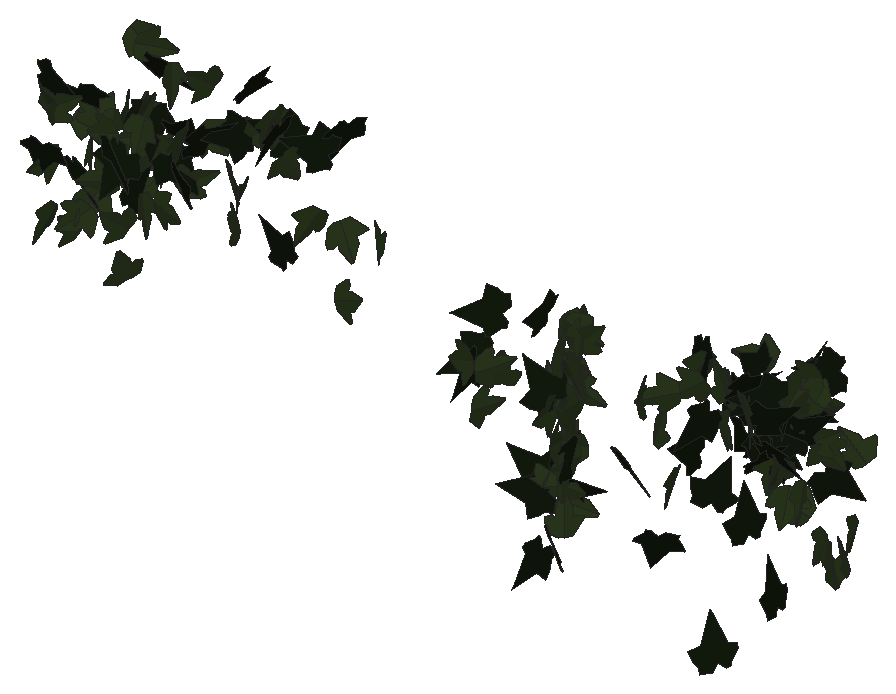
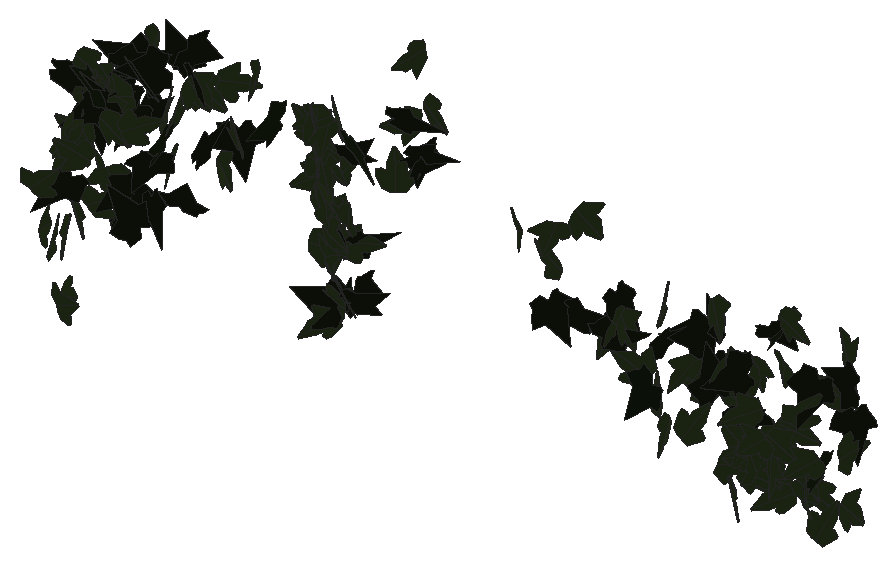
# SketchUp Ruby script. Lengths in inches.
U = 1.inch
M = Sketchup.active_model
def pt(a) = Geom::Point3d.new(a.map { |v| v * U })
def face(e, loops, mat)
  f = e.add_face(loops[0].map { |a| pt(a) })
  loops[1..].each { |l| e.add_face(l.map { |a| pt(a) }).erase! }
  f.material = f.back_material = mat if mat
  f
end
# faces: each face lists its corners as indices into pts; further lists are holes
def faces(e, pts, list, mat = nil) = list.each { |f| face(e, (f[0].is_a?(Array) ? f : [f]).map { |l| l.map { |i| pts[i] } }, mat) }
# xy, xz, yz: faces in a plane at the given z, y or x. An outline is a flat list of corners, or four numbers for a rectangle; further outlines are holes
def ring(l) = l.size == 4 ? [[l[0], l[1]], [l[2], l[1]], [l[2], l[3]], [l[0], l[3]]] : l.each_slice(2).to_a
def flat(e, list, mat, &to3) = list.each { |f| face(e, (f[0].is_a?(Array) ? f : [f]).map { |l| ring(l).map { |u, v| to3.(u, v) } }, mat) }
def xy(e, z, list, mat = nil) = flat(e, list, mat) { |x, y| [x, y, z] }
def xz(e, y, list, mat = nil) = flat(e, list, mat) { |x, z| [x, y, z] }
def yz(e, x, list, mat = nil) = flat(e, list, mat) { |y, z| [x, y, z] }
def lines(e, pts, list) = list.each { |a, b| e.add_line(pt(pts[a]), pt(pts[b])) }
# prism: a flat outline (further loops are holes) pulled along v
def prism(e, loops, v, mat = nil)
  f = face(e, loops, mat); d = Geom::Vector3d.new(v.map { |x| x * U })
  f.pushpull(f.normal.samedirection?(d) ? d.length : -d.length)
end
def box(e, o, s, mat = nil) = prism(e, [[o, [o[0] + s[0], o[1], o[2]], [o[0] + s[0], o[1] + s[1], o[2]], [o[0], o[1] + s[1], o[2]]]], [0, 0, s[2]], mat)
def at(x, y, z, deg = 0) = Geom::Transformation.translation(pt([x, y, z])) * Geom::Transformation.rotation(ORIGIN, Z_AXIS, deg.degrees)
def axes(o, x, y, z) = Geom::Transformation.new([*x, 0, *y, 0, *z, 0, *pt(o).to_a, 1])
def part(name) = M.definitions.add(name)
# library, detail: a bought-in or finely detailed component or shape, given as its bounding box
def library(name, o, s) = part(name).tap { |d| box(d.entities, o, s) }
def detail(e, o, s) = box(e.add_group.entities, o, s)
def put(e, d, t, mat = nil) = e.add_instance(d, t).tap { |i| i.material = mat if mat }
def group(e, t, mat = nil) = e.add_group.tap { |g| g.transformation = t; g.material = mat if mat }.entities
root = M.entities
M.materials.add("efeu1").color = [18, 25, 13]
M.materials.add("efeu2").color = [43, 57, 29]
c1 = part("ivyleaf_10")
p = [[0,0.5,-0.03],[-0.0625,2.02,-0.43],[-0.19,2.01,-0.46],[-0.54,1.05,-0.29],[-0.52,0.625,-0.18],[-0.83,0.76,-0.28],
  [-1.16,0.64,-0.33],[-1.15,0.33,-0.24],[-0.77,-0.39,0.02],[-0.3,-0.51,0.16],[0.04,-0.48,0.23],[-0.02,2.01,-0.4375],
  [-0.06,2.01,-0.43],[0.04,-0.49,0.23],[0.67,-0.49,0.14],[1.38,0.36,-0.2],[1.375,0.51,-0.24],[0.81,0.65,-0.19],
  [0.62,0.59,-0.15],[0.6,1.09,-0.28],[0.5,1.23,-0.31]]
faces(c1.entities,p,[[0,1,2,3,4,5,6,7,8,9,10],[11,12,0,13,14,15,16,17,18,19,20]],"efeu2")
c2 = part("ivyleaf_9")
p = [[1.54,2.16,1.25],[1.36,2.04,1.19],[-0.21,0.99,0.68],[-0.71,1.11,0.82],[-0.85,0.86,0.67],[-0.8,0.17,0.21],
  [-0.9,-0.01,0.1],[-0.67,-0.16,-0.02],[-0.08,-0.08,-0.05],[-0.03,-0.6,-0.4],[0.65,-0.88,-0.66],[0.83,-0.6,-0.49],
  [1.29,-0.42,-0.43],[1.8125,-0.07,-0.26],[1.21,0.44,0.15]]
faces(c2.entities,p,[[0,1,2,3,4,5,6,7,8,9,10,11,12,13,14]],"efeu1")
put(root,c1,axes([26.62,223.76,193.08],[-0.0284,0.01779,-0.49888],[-0.14979,-0.47696,-0.00849],[-0.47619,0.14897,0.03242]))
put(root,c2,axes([26.15,223.96,195.55],[0.24856,-0.04735,-0.43125],[0.42245,0.13954,0.22817],[0.09874,-0.47779,0.10937]))
put(root,c1,axes([26.58,223.71,191.38],[0.07742,-0.36257,0.33548],[0.07667,-0.32664,-0.37071],[0.48798,0.10884,0.00502]))
put(root,c1,axes([26.34,225.81,192.59],[0.13191,-0.08299,0.47509],[0.38107,-0.28397,-0.15541],[0.29561,0.40308,-0.01167]))
put(root,c1,axes([26.45,225.41,193.65],[0.21774,0.18874,0.40861],[0.30341,0.27373,-0.28812],[-0.33246,0.37343,0.00467]))
put(root,c1,axes([26.47,227.7,195.32],[0.28749,0.11923,0.39132],[0.36164,0.1495,-0.31124],[-0.19122,0.46199,-0.00028]))
put(root,c2,axes([26.93,222.92,193.96],[0.29364,0.23583,-0.32887],[-0.27196,-0.1859,-0.37614],[-0.29968,0.39978,0.0191]))
put(root,c1,axes([27.04,224.35,190.71],[-0.1528,-0.2963,-0.37264],[-0.13276,-0.34932,0.33219],[-0.45719,0.20047,0.02808]))
put(root,c1,axes([26.73,223.62,194.81],[-0.25829,-0.13735,0.40549],[0.35117,0.20289,0.29242],[-0.24487,0.43585,-0.00834]))
put(root,c1,axes([27.13,226.38,193.78],[0.08231,-0.36855,-0.32771],[-0.08156,0.3175,-0.37755],[0.48639,0.11561,-0.00785]))
put(root,c2,axes([26.97,224.32,192.74],[0.34112,-0.36522,0.01576],[0.0134,-0.00904,-0.49974],[0.36532,0.34137,0.00362]))
put(root,c2,axes([27.3125,224.11,195.39],[0.39415,0.29152,-0.09829],[-0.07931,-0.05806,-0.49024],[-0.29725,0.40205,0.00047]))
put(root,c1,axes([27.53,224.75,194.38],[0.22778,0.33838,0.28916],[-0.15531,-0.24398,0.40786],[0.41713,-0.27562,-0.00604]))
put(root,c1,axes([27.64,223.89,191.63],[0.33009,0.08195,-0.36651],[-0.36287,-0.05617,-0.33937],[-0.0968,0.49003,0.02239]))
put(root,c1,axes([27.28,222.7,195.51],[-0.27672,0.06796,0.41086],[0.38661,-0.14143,0.28378],[0.15479,0.47474,0.02573]))
put(root,c1,axes([27.29,225.6,192.34],[0.09866,0.14487,0.46827],[0.27252,0.38083,-0.17523],[-0.40743,0.2898,-0.00381]))
put(root,c1,axes([27.41,226.92,195.62],[0.0891,0.08984,0.48372],[0.212,0.4366,-0.12014],[-0.44398,0.22651,0.03971]))
put(root,c1,axes([27.74,224.29,192.03],[0.28153,0.30283,-0.28112],[-0.20739,-0.19066,-0.41308],[-0.35739,0.3492,0.01825]))
put(root,c1,axes([28.02,226.3125,193.18],[0.15422,0.04089,-0.47386],[-0.47392,-0.02887,-0.15673],[-0.04018,0.49749,0.02985]))
put(root,c1,axes([27.72,226.32,193.34],[0.0667,0.42113,-0.26115],[0.04213,0.25773,0.42638],[0.49374,-0.07889,-0.0011]))
put(root,c1,axes([28.21,226.27,194.11],[-0.01737,0.40647,-0.29065],[0.00094,-0.2908,-0.40674],[-0.4997,-0.01468,0.00934]))
put(root,c1,axes([28.66,224.4,193.08],[-0.23568,-0.18544,0.40008],[-0.31994,-0.24028,-0.29984],[0.30347,-0.39734,-0.0054]))
put(root,c1,axes([28.73,223.69,193.18],[-0.10709,-0.05814,0.48492],[-0.41611,-0.24906,-0.12175],[0.2557,-0.42964,0.00496]))
put(root,c1,axes([28.64,226.32,192.53],[0.2734,-0.36018,-0.21337],[-0.12078,0.17613,-0.45209],[0.40083,0.29875,0.0093]))
put(root,c1,axes([28.62,225.48,193.18],[0.02432,0.08357,-0.49237],[0.19315,0.45301,0.08643],[0.46054,-0.19441,-0.01025]))
put(root,c1,axes([29,226.13,193.03],[0.11589,0.11121,-0.4735],[-0.33248,-0.33716,-0.16057],[-0.355,0.35207,-0.0042]))
put(root,c2,axes([28.74,225.58,194.55],[-0.2933,-0.32037,-0.24767],[0.17032,0.17985,-0.43433],[0.36738,-0.33915,0.00363]))
put(root,c2,axes([28.56,225.8125,195.9375],[0.45319,-0.05575,0.20375],[0.20116,-0.03326,-0.45654],[0.06446,0.49577,-0.00771]))
put(root,c1,axes([28.83,223.68,195.19],[0.42507,-0.15942,0.20952],[0.19549,-0.0754,-0.45398],[0.17634,0.46787,-0.00177]))
put(root,c1,axes([29.18,227.66,194.68],[-0.14249,-0.24996,-0.40892],[-0.20497,-0.35385,0.28771],[-0.43323,0.24962,-0.00163]))
put(root,c1,axes([29.2,224.58,194.89],[0.07486,-0.16035,0.46764],[-0.23222,0.40614,0.17644],[-0.43643,-0.2436,-0.01367]))
put(root,c1,axes([29.39,225.38,193.61],[0.29267,-0.08357,-0.39669],[-0.36996,0.145,-0.30349],[0.16577,0.47116,0.02304]))
put(root,c2,axes([29.13,224.09,192.4],[-0.19206,0.31082,0.34132],[0.1802,-0.28988,0.36537],[0.42502,0.26336,-0.00067]))
put(root,c1,axes([29.15,224.36,192.47],[0.36808,-0.0235,-0.33759],[0.33789,-0.00205,0.36855],[-0.01871,-0.49944,0.01437]))
put(root,c1,axes([29.4,225.67,196],[-0.03051,0.46685,-0.17641],[0.01122,-0.17605,-0.46785],[-0.49894,-0.0325,0.00027]))
put(root,c1,axes([29.85,222.3125,195.68],[0.18102,-0.08307,-0.45862],[-0.4215,0.1808,-0.19912],[0.19892,0.4587,-0.00457]))
put(root,c1,axes([29.7,223.14,192.25],[-0.17859,-0.24892,-0.39515],[-0.22572,-0.32435,0.30634],[-0.40885,0.2878,0.00348]))
put(root,c1,axes([29.66,223.97,195.13],[0.49312,-0.08109,-0.01608],[-0.01551,0.00484,-0.49974],[0.0812,0.49336,0.00226]))
put(root,c1,axes([29.8125,223.07,190.75],[-0.21269,-0.41069,-0.19],[-0.08712,-0.16885,0.46249],[-0.44404,0.22984,0.00027]))
put(root,c1,axes([30.21,223.38,193.08],[-0.11617,0.47045,-0.1232],[0.03003,-0.11949,-0.48458],[-0.48539,-0.11999,-0.00049]))
put(root,c2,axes([30.03,222.21,195.34],[0.23477,-0.43236,0.08915],[0.04009,-0.07968,-0.49198],[0.43963,0.23815,-0.00275]))
put(root,c2,axes([30.48,222.21,195.19],[-0.39779,-0.30206,-0.02288],[0.0212,0.00992,-0.49945],[0.30218,-0.39833,0.00491]))
put(root,c2,axes([30.1875,225.09,194.47],[0.49966,0.01557,-0.00997],[0.00951,0.01506,0.49968],[0.01586,-0.49953,0.01475]))
put(root,c2,axes([30.89,227.16,195.34],[0.12961,0.38678,0.28914],[0.09464,0.27322,-0.40791],[-0.47355,0.16046,-0.00238]))
put(root,c2,axes([30.94,223.71,194.66],[0.02144,-0.28482,-0.41039],[-0.03384,0.40899,-0.28562],[0.49839,0.04002,-0.00173]))
put(root,c1,axes([30.84,223.35,193.22],[-0.04714,0.02418,-0.49719],[0.42355,-0.26041,-0.05282],[-0.2615,-0.42615,0.00406]))
put(root,c1,axes([31.19,224.96,194.95],[0.0858,0.36591,0.32977],[0.08116,0.31966,-0.37581],[-0.48585,0.11802,-0.00454]))
put(root,c1,axes([31.34,225.88,193.34],[-0.36488,0.34077,0.02714],[-0.02135,0.0169,-0.49926],[-0.34118,-0.3655,0.00222]))
put(root,c1,axes([31.2,224.03,193.73],[-0.15654,-0.17991,0.43947],[0.2864,0.33333,0.23847],[-0.37878,0.32638,-0.00131]))
put(root,c1,axes([31.6875,223.25,195.86],[0.09218,-0.49118,-0.01556],[-0.00321,0.01523,-0.49976],[0.49142,0.09223,-0.00034]))
put(root,c2,axes([31.62,223.79,195.3],[0.03251,0.36527,-0.33989],[-0.02699,0.34139,0.36431],[0.49821,-0.00534,0.04191]))
put(root,c2,axes([32.27,225.23,195.25],[0.04968,-0.35318,-0.35043],[0.08062,-0.3418,0.35591],[-0.49095,-0.09186,0.02299]))
put(root,c2,axes([32.07,222.74,194.52],[-0.02639,-0.07411,0.49377],[0.2081,-0.4511,-0.05658],[0.45387,0.20252,0.05466]))
put(root,c1,axes([32.16,225.96,194.81],[-0.20519,-0.26163,0.37343],[0.23032,0.29394,0.33249],[-0.39351,0.30846,-0.00011]))
put(root,c1,axes([32.33,225.07,193.21],[0.11461,-0.35333,-0.33469],[0.09839,-0.31993,0.37144],[-0.47664,-0.151,-0.00381]))
put(root,c1,axes([33.08,225.57,195.9],[0.07329,-0.46972,0.15491],[0.04221,-0.15008,-0.47507],[0.49279,0.08272,0.01766]))
put(root,c2,axes([33.68,225.72,195.27],[-0.15169,0.03844,0.47488],[-0.47006,0.06916,-0.15574],[-0.07766,-0.4937,0.01515]))
put(root,c1,axes([33.3,225.78,195.91],[-0.00775,0.34917,-0.3578],[-0.00742,-0.35788,-0.34909],[-0.49988,-0.0001,0.01073]))
put(root,c2,axes([33.93,224.82,196.17],[-0.21053,0.35683,-0.2799],[0.12905,-0.2487,-0.41412],[-0.43477,-0.24662,0.01262]))
put(root,c1,axes([34.1,224.89,195.17],[-0.17733,-0.39408,-0.2515],[0.10974,0.22638,-0.4321],[0.45444,-0.20844,0.0062]))
put(root,c1,axes([34.39,222.3,194.17],[-0.25718,0.3059,0.30047],[0.19285,-0.23042,0.39964],[0.38297,0.32145,0.00053]))
put(root,c2,axes([35.04,225.56,195.4],[-0.22892,0.04265,0.44247],[-0.43705,0.06925,-0.23279],[-0.08114,-0.49334,0.00558]))
put(root,c2,axes([35.28,226.22,196.07],[-0.04527,0.36959,-0.33369],[0.05326,-0.32955,-0.37224],[-0.49509,-0.06925,-0.00953]))
put(root,c2,axes([35.59,223.03,193.35],[0.03167,-0.05461,0.496],[-0.34113,0.36035,0.06145],[-0.36418,-0.34229,-0.01444]))
put(root,c1,axes([37.73,221.71,196.01],[-0.12506,-0.37647,0.30435],[-0.05999,-0.29987,-0.39558],[0.48038,-0.13546,0.02983]))
put(root,c1,axes([38.35,222.16,195.6],[0.28487,0.38413,0.14592],[0.08768,0.11664,-0.47823],[-0.40145,0.29806,-0.00091]))
put(root,c1,axes([38.92,221.42,193.86],[0.15555,-0.10273,-0.46395],[0.40968,-0.21835,0.1857],[-0.24076,-0.43791,0.01624]))
put(root,c1,axes([39.52,222.38,195.1875],[0.22812,-0.13112,0.42517],[-0.37309,0.20394,0.26307],[-0.24241,-0.43728,-0.00479]))
put(root,c2,axes([44.99,220.28,194.76],[-0.35629,-0.19256,0.29322],[-0.25127,-0.15155,-0.40484],[0.24479,-0.43584,0.01122]))
put(root,c2,axes([45.26,220.61,196.01],[-0.35669,0.04406,0.34761],[-0.34883,0.00215,-0.35821],[-0.03306,-0.49805,0.0292]))
put(root,c2,axes([44.83,220.03,194.625],[-0.01324,-0.0066,-0.49978],[0.30691,-0.39471,-0.00292],[-0.3945,-0.30685,0.01451]))
put(root,c1,axes([45.59,218.71,195.45],[0.17876,-0.12563,-0.44974],[-0.37244,0.25211,-0.21846],[0.28166,0.4131,-0.00345]))
put(root,c1,axes([45.32,220.6,193.95],[-0.41714,-0.27564,0.00375],[0.00507,-0.00087,0.49997],[-0.27562,0.41716,0.00352]))
put(root,c2,axes([45.9,221.82,190.39],[-0.39497,-0.23526,-0.1966],[-0.15948,-0.11618,0.45942],[-0.26185,0.42562,0.01673]))
put(root,c2,axes([45.9,221.9,195.64],[-0.31008,0.36449,0.14492],[-0.09262,0.11147,-0.47854],[-0.38115,-0.32361,-0.00161]))
put(root,c1,axes([46.01,221.95,192.98],[0.45059,-0.10071,0.1919],[-0.18472,0.05309,0.46159],[-0.11335,-0.48687,0.01064]))
put(root,c1,axes([45.86,219.125,195.07],[0.03033,0.02346,-0.49853],[0.31445,0.38695,0.03734],[0.38756,-0.31579,0.00872]))
put(root,c2,axes([46.03,221.9,190.43],[-0.21396,0.37577,0.25103],[0.12075,-0.22011,0.4324],[0.43548,0.24566,0.00344]))
put(root,c1,axes([46.55,222.05,192.58],[0.06146,-0.04719,-0.49396],[-0.39558,0.29583,-0.07748],[0.29957,0.40032,-0.00097]))
put(root,c1,axes([46.64,222.08,191.74],[0.26564,-0.06568,0.41847],[-0.40573,0.1025,0.27364],[-0.12173,-0.48495,0.00116]))
put(root,c1,axes([46.87,222,193.1875],[0.23027,-0.06528,0.43899],[-0.41404,0.14651,0.23897],[-0.15983,-0.47357,0.01342]))
put(root,c1,axes([46.29,222.02,190.27],[0.00871,-0.00142,-0.49992],[0.46868,-0.17398,0.00866],[-0.17397,-0.46875,-0.0017]))
put(root,c1,axes([46.63,222.04,193.23],[0.1694,-0.45812,0.10692],[-0.03721,0.10024,0.48843],[-0.46896,-0.17343,-0.00013]))
put(root,c1,axes([46.51,222.05,189.7],[0.10212,0.17996,0.45518],[0.22467,0.39587,-0.20692],[-0.43485,0.24679,-0.00001]))
put(root,c1,axes([47.14,221.84,191.88],[0.04662,0.01734,-0.49752],[-0.49005,0.08957,-0.0428],[0.08765,0.49161,0.02535]))
put(root,c2,axes([46.37,222.03,190.2],[0.29568,0.19988,-0.35017],[0.28911,0.19758,0.3569],[0.28105,-0.41353,0.00127]))
put(root,c1,axes([46.74,221.94,195.7],[0.05055,0.49684,0.02433],[0.00031,0.02442,-0.4994],[-0.49744,0.05051,0.00216]))
put(root,c1,axes([47.02,222.09,195.3],[0.19474,-0.32018,-0.331],[-0.14729,0.29719,-0.37414],[0.43633,0.24323,0.02143]))
put(root,c1,axes([47.17,220.37,191.21],[-0.04612,0.01161,0.49773],[-0.28028,-0.41374,-0.01632],[0.41148,-0.28051,0.04467]))
put(root,c1,axes([47.15,221.68,194.6],[0.35672,-0.04526,-0.34742],[-0.34535,0.0381,-0.35956],[0.05902,0.49649,-0.00408]))
put(root,c2,axes([47.2,220.27,191.08],[-0.13983,-0.35775,-0.32009],[-0.09201,-0.30724,0.38359],[-0.47115,0.16618,0.02009]))
put(root,c2,axes([47.26,220.48,194.07],[-0.4239,-0.25638,-0.06764],[-0.05554,-0.03887,0.49538],[-0.25927,0.4275,0.00448]))
put(root,c1,axes([47.22,221.69,194.52],[-0.41814,-0.02099,0.27334],[-0.27207,-0.02949,-0.41846],[0.03369,-0.49869,0.01324]))
put(root,c1,axes([47.24,220.59,192.42],[-0.07993,0.12352,0.47786],[-0.29827,0.37361,-0.14646],[-0.39325,-0.30848,0.01396]))
put(root,c1,axes([47.21,221.04,189.58],[0.18098,0.45598,-0.09657],[0.03159,0.09136,0.49057],[0.46503,-0.18367,0.00426]))
put(root,c1,axes([47.28,221.84,195.99],[0.27852,-0.39665,-0.12286],[-0.05711,0.10995,-0.48441],[0.4113,0.28386,0.01594]))
put(root,c1,axes([47.26,220.9,191.51],[-0.06653,-0.49552,0.00572],[0.11447,-0.02098,-0.48627],[0.48215,-0.06339,0.11623]))
put(root,c1,axes([47.26,221.43,191.67],[-0.01171,0.07785,0.49376],[0.12569,-0.47757,0.07828],[0.4838,0.12596,-0.00838]))
put(root,c1,axes([47.27,220.4375,193.65],[0.0094,-0.02148,-0.49945],[-0.03186,-0.49855,0.02084],[-0.4989,0.03143,-0.01074]))
put(root,c1,axes([47.11,220.85,195.0625],[0.27461,-0.31634,-0.27297],[0.17761,-0.2073,0.41891],[-0.37821,-0.32704,-0.00149]))
put(root,c1,axes([47.22,221.77,193.4],[-0.04186,0.08646,0.49069],[0.21621,-0.44048,0.09606],[0.44889,0.22023,-0.00051]))
put(root,c1,axes([47.26,221.24,192.69],[-0.44175,0.10252,0.2106],[0.20523,-0.04725,0.45349],[0.11288,0.48709,-0.00033]))
put(root,c1,axes([47.31,221.84,195.77],[-0.03509,-0.45809,0.19729],[0.15363,-0.19809,-0.43262],[0.47452,0.03025,0.15466]))
put(root,c1,axes([47.26,221.29,194.67],[-0.43093,0.16982,-0.18832],[0.17644,-0.06589,-0.46317],[-0.18212,-0.46564,-0.00314]))
put(root,c2,axes([47.35,219.84,189.42],[0.02161,-0.02121,-0.49908],[0.23735,-0.43912,0.02894],[-0.43954,-0.23817,-0.00891]))
put(root,c2,axes([47.25,220.82,191.57],[-0.23565,0.2942,0.3285],[0.19011,-0.26831,0.37666],[0.3979,0.30242,0.0146]))
put(root,c1,axes([47.1,221.62,195.83],[-0.25153,-0.03007,-0.43108],[0.43044,0.02654,-0.25301],[0.0381,-0.49839,0.01254]))
put(root,c1,axes([47.26,221.35,194.86],[-0.3316,0.24207,-0.28538],[0.23422,-0.16313,-0.41052],[-0.29186,-0.40594,-0.0052]))
put(root,c2,axes([47.21,220.57,189.18],[0.07961,-0.17725,0.4607],[0.16345,-0.43086,-0.19401],[0.46578,0.18149,-0.01066]))
put(root,c1,axes([47.23,221.54,193.9375],[-0.25372,-0.06223,-0.42633],[0.42347,0.05516,-0.26006],[0.0794,-0.49304,0.02471]))
put(root,c1,axes([47.32,221.66,195.33],[-0.3166,-0.19284,0.33553],[0.29544,0.15956,0.37048],[-0.24996,0.43284,0.01291]))
put(root,c1,axes([47.66,216.62,195.55],[-0.01957,-0.0773,-0.4936],[0.18973,0.45583,-0.0789],[0.46219,-0.19039,0.01149]))
put(root,c1,axes([50.44,221.27,193.6],[0.41595,-0.27746,-0.00053],[0.0041,0.0052,0.49996],[-0.27743,-0.41592,0.0066]))
put(root,c1,axes([50.74,220.1,195.31],[-0.05323,0.09573,0.48785],[-0.30852,0.37838,-0.10791],[-0.38985,-0.31252,0.01879]))
put(root,c2,axes([50.4,219.57,193.69],[0.41393,-0.27684,0.04491],[0.04172,-0.01839,-0.49792],[0.27734,0.41596,0.00788]))
put(root,c1,axes([51.13,220.97,195.31],[-0.05899,-0.0394,0.49494],[-0.26292,-0.42033,-0.06479],[0.42118,-0.26791,0.02888]))
put(root,c1,axes([51.19,222.41,195.79],[-0.06719,-0.41501,0.27066],[-0.04022,-0.26766,-0.4204],[0.49383,-0.07827,0.00259]))
put(root,c2,axes([51.34,224.03,192.78],[0.18546,0.054,-0.46118],[-0.4575,-0.06366,-0.19143],[-0.07939,0.49298,0.0258]))
put(root,c1,axes([51.46,221.8,195.39],[-0.23881,-0.16003,0.4091],[-0.3331,-0.23759,-0.28739],[0.28638,-0.4098,0.00687]))
put(root,c1,axes([51.18,221.11,192.67],[0.18217,-0.4321,0.17349],[0.07828,-0.15522,-0.4688],[0.459,0.19797,0.0111]))
put(root,c2,axes([51.0625,222.52,196.16],[-0.26259,-0.00419,-0.42547],[0.42546,0.00366,-0.26262],[0.00531,-0.49997,0.00164]))
put(root,c2,axes([51.43,221.8,193.15],[-0.06364,-0.03165,0.49492],[-0.22271,-0.44401,-0.05703],[0.44311,-0.22771,0.04242]))
put(root,c1,axes([51.5,222.91,194.68],[-0.15246,0.47496,0.03425],[0.00658,-0.03386,0.49881],[0.47614,0.15254,0.00407]))
put(root,c2,axes([51.17,223.72,194.55],[0.33998,-0.36633,0.01455],[0.01347,-0.00735,-0.49976],[0.36637,0.34022,0.00487]))
put(root,c1,axes([51.6,222.75,193.625],[-0.25785,0.36257,0.22815],[-0.13353,0.185,-0.44491],[-0.40704,-0.29037,0.00143]))
put(root,c1,axes([51.76,224.53,195.1],[0.10226,0.14017,0.46893],[-0.27312,-0.38119,0.1735],[0.40614,-0.29163,-0.00139]))
put(root,c2,axes([51.38,224,194.09],[-0.08434,-0.34113,-0.35569],[0.0902,0.34408,-0.35139],[0.48451,-0.12344,0.0035]))
put(root,c2,axes([51.53,224.42,192.04],[0.26294,0.4245,0.02576],[-0.01585,-0.02049,0.49933],[0.42498,-0.2634,0.00268]))
put(root,c1,axes([51.9,222.81,194.64],[-0.2858,0.40978,0.01989],[0.00662,-0.01964,0.49957],[0.41021,0.28582,0.0058]))
put(root,c2,axes([52.375,224.35,192.04],[0.09352,-0.48915,0.04457],[0.00084,0.04553,0.49792],[-0.49118,-0.09305,0.00934]))
put(root,c2,axes([52.09,223.9375,192.92],[-0.02682,-0.09871,-0.48943],[0.19105,0.4508,-0.10139],[0.46128,-0.19245,0.01354]))
put(root,c2,axes([52.57,218.62,192.21],[0.22205,0.33468,-0.29779],[-0.17383,-0.24195,-0.40155],[-0.41289,0.28186,0.00891]))
put(root,c2,axes([52.8,222.87,195.77],[-0.18462,0.26695,0.38033],[-0.24345,0.29302,-0.32384],[-0.39579,-0.30476,0.02178]))
put(root,c2,axes([52.89,220.44,195.52],[-0.01576,-0.00396,-0.49974],[0.18354,-0.46509,-0.00211],[-0.46483,-0.18351,0.01611]))
put(root,c2,axes([52.74,221.875,195.59],[0.03796,0.357,-0.34801],[-0.00014,0.34903,0.35802],[0.49856,-0.02708,0.0266]))
put(root,c1,axes([52.71,225.46,194.31],[0.24846,0.15298,-0.40603],[0.35398,0.19912,0.29163],[0.25093,-0.43237,-0.00936]))
put(root,c1,axes([53.37,223.54,194.34],[0.17229,-0.04278,-0.46742],[-0.42347,0.20059,-0.17445],[0.20245,0.456,0.03288]))
put(root,c1,axes([53.8125,224.75,194.32],[-0.28276,0.22173,-0.34768],[-0.29096,0.19146,0.35873],[0.29222,0.40519,0.02076]))
put(root,c2,axes([53.3,221.76,195.52],[-0.06718,0.02827,-0.49466],[0.47618,-0.13424,-0.07234],[-0.1369,-0.48081,-0.00889]))
put(root,c2,axes([53.9,222.27,195.47],[-0.2104,-0.08773,0.44501],[-0.41273,-0.16642,-0.22794],[0.18812,-0.46326,-0.00239]))
put(root,c1,axes([53.95,223.37,191.43],[0.19114,0.19296,0.4198],[-0.3547,-0.22983,0.26715],[0.29606,-0.39993,0.04903]))
put(root,c2,axes([53.5,222.66,193.75],[-0.07051,0.21886,0.44399],[0.13624,-0.42257,0.22994],[0.47589,0.1534,-0.00005]))
put(root,c1,axes([53.625,221.1,195.91],[-0.3512,0.31401,-0.1675],[0.12132,-0.1156,-0.47108],[-0.33457,-0.37153,0.005]))
put(root,c1,axes([54.01,224.6,188.98],[-0.13635,0.16019,-0.45359],[-0.31583,0.32581,0.21],[0.36285,0.34378,0.01234]))
put(root,c2,axes([53.6875,223.57,195.33],[-0.20152,0.45759,-0.00104],[-0.01279,-0.00449,0.49982],[0.45741,0.20147,0.01352]))
put(root,c1,axes([53.69,224.46,194.2],[-0.05753,-0.15457,-0.47202],[0.15202,0.44689,-0.16487],[0.47284,-0.16248,-0.00442]))
put(root,c1,axes([54.05,224.8,188.75],[0.24241,-0.02576,0.43655],[-0.43531,0.0334,0.2437],[-0.04171,-0.49822,-0.00623]))
put(root,c2,axes([53.79,221.62,193.83],[0.20545,0.43048,0.14993],[0.0531,0.14073,-0.47684],[-0.45274,0.21185,0.01211]))
put(root,c1,axes([53.5,222.55,194.71],[0.11001,0.04033,0.48608],[0.42571,0.23526,-0.11587],[-0.23806,0.43935,0.01742]))
put(root,c2,axes([53.65,223.28,194.78],[0.02341,0.04755,-0.49718],[0.09373,0.48847,0.05113],[0.49058,-0.09559,0.01396]))
put(root,c1,axes([53.93,223.31,195.5],[0.12414,0.34746,-0.33744],[-0.14087,-0.30738,-0.36834],[-0.46341,0.18652,0.02157]))
put(root,c1,axes([53.9,222.78,192.22],[0.33978,0.35354,-0.09779],[-0.06748,-0.07078,-0.49034],[-0.36055,0.34641,-0.00039]))
put(root,c1,axes([53.94,222.91,194.3],[-0.42791,-0.24494,0.08305],[0.07708,0.03248,0.49295],[-0.24688,0.43468,0.00996]))
put(root,c2,axes([54.11,223.04,194.49],[0.09492,0.46323,-0.16252],[-0.03917,-0.15785,-0.47281],[-0.48934,0.10249,0.00632]))
put(root,c1,axes([54.36,223.36,195.92],[0.21326,-0.00863,-0.45216],[-0.43834,0.11903,-0.20902],[0.11125,0.48555,0.0432]))
put(root,c1,axes([54.32,223.58,195],[0.24311,0.18378,0.39639],[-0.32113,-0.23244,0.30471],[0.29627,-0.40274,0.00502]))
put(root,c1,axes([54.14,222.89,194.9],[-0.00144,0.21152,0.45306],[-0.14352,0.43382,-0.20299],[-0.47896,-0.13063,0.05946]))
put(root,c2,axes([54.09,222.75,194.36],[-0.22358,-0.43192,0.11601],[-0.05485,-0.10224,-0.48635],[0.44385,-0.2302,-0.00167]))
put(root,c1,axes([54.23,221.99,193.6],[-0.26305,-0.39155,0.16582],[-0.08262,-0.14421,-0.47157],[0.41711,-0.27549,0.01117]))
put(root,c2,axes([54.58,224.16,195.87],[-0.15492,-0.13431,-0.45603],[-0.36755,-0.27036,0.20448],[-0.30151,0.39858,-0.01497]))
put(root,c2,axes([53.93,221.42,195.11],[0.06761,-0.04411,0.49344],[0.49262,0.05874,-0.06225],[-0.05248,0.49457,0.0514]))
put(root,c2,axes([54.11,221.49,194.38],[0.49888,0.01379,0.0304],[0.0304,0.00015,-0.49907],[-0.01377,0.49981,-0.00068]))
put(root,c1,axes([54.58,225.26,192.64],[0.31805,0.20455,0.32712],[-0.2979,-0.13919,0.37667],[0.24516,-0.4345,0.03333]))
put(root,c1,axes([54.12,223.72,193.61],[-0.27683,-0.11123,0.40124],[0.37103,0.15275,0.29834],[-0.18895,0.46292,-0.00203]))
put(root,c1,axes([54.22,221.94,193.64],[0.01312,-0.0336,0.4987],[0.29953,-0.39884,-0.03475],[0.40014,0.29966,0.00966]))
put(root,c1,axes([54.31,223.93,193.37],[-0.29227,-0.29934,-0.27382],[0.21362,0.17335,-0.41751],[0.34489,-0.36103,0.02656]))
put(root,c2,axes([54.35,218.83,193.93],[-0.33339,-0.02975,0.37143],[0.37076,-0.07632,0.32667],[0.03725,0.49324,0.07295]))
put(root,c2,axes([54.13,222.66,194.32],[0.04369,-0.06053,0.4944],[0.49712,0.03629,-0.03949],[-0.0311,0.49499,0.06335]))
put(root,c2,axes([54.28,224.09,192.47],[0.02218,-0.1243,-0.48379],[0.03711,0.48334,-0.12249],[0.49813,-0.03048,0.03067]))
put(root,c2,axes([54.73,218.5625,189.01],[-0.49422,-0.04855,0.05823],[0.05833,0.00178,0.49658],[-0.04842,0.49763,0.0039]))
put(root,c1,axes([54.46,222.67,192.63],[0.3949,-0.24651,0.18245],[0.15021,-0.10386,-0.46546],[0.26738,0.42243,-0.00797]))
put(root,c2,axes([54.67,220.04,192.51],[-0.22276,-0.34714,0.28262],[0.22307,0.18761,0.40625],[-0.38809,0.30708,0.07129]))
put(root,c2,axes([54.86,221.09,189.77],[-0.06428,-0.3998,0.29331],[0.12308,0.27364,0.39997],[-0.48033,0.12361,0.06324]))
put(root,c1,axes([54.92,223.07,190.97],[0.36721,-0.29846,-0.1615],[-0.11353,0.11619,-0.47287],[0.3198,0.38395,0.01757]))
put(root,c1,axes([55.02,223.26,190.39],[-0.31784,0.32587,0.20684],[-0.14612,0.14642,-0.45521],[-0.35725,-0.34981,0.00215]))
put(root,c1,axes([55.05,223.97,189.875],[-0.32426,0.36939,0.09166],[0.05516,-0.07354,0.49148],[0.37658,0.32885,0.00694]))
put(root,c1,axes([54.95,224.4375,190.76],[0.05706,-0.13785,0.47722],[0.3025,-0.37138,-0.14344],[0.39401,0.30509,0.04102]))
